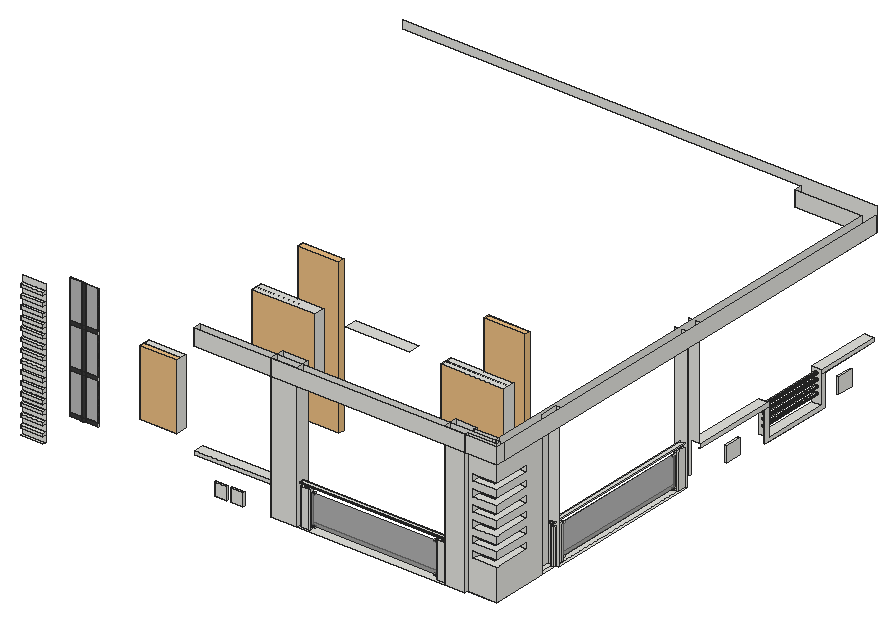
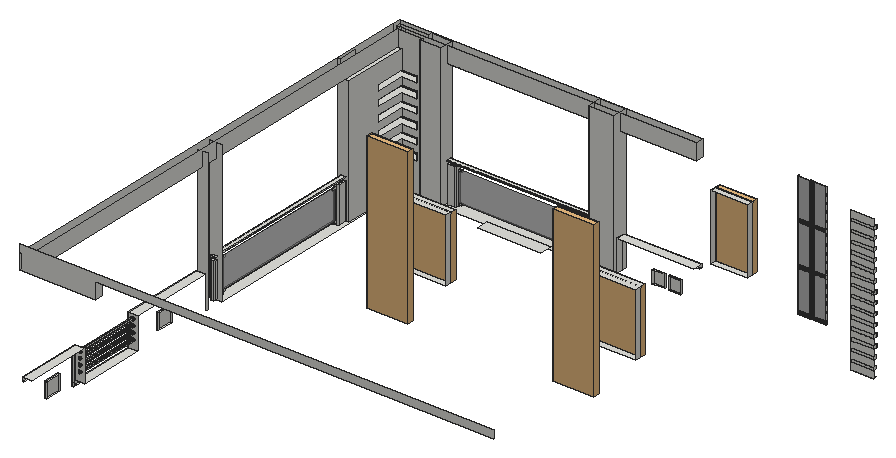
# SketchUp Ruby script. Lengths in inches.
U = 1.inch
M = Sketchup.active_model
def pt(a) = Geom::Point3d.new(a.map { |v| v * U })
def face(e, loops, mat)
  f = e.add_face(loops[0].map { |a| pt(a) })
  loops[1..].each { |l| e.add_face(l.map { |a| pt(a) }).erase! }
  f.material = f.back_material = mat if mat
  f
end
# faces: each face lists its corners as indices into pts; further lists are holes
def faces(e, pts, list, mat = nil) = list.each { |f| face(e, (f[0].is_a?(Array) ? f : [f]).map { |l| l.map { |i| pts[i] } }, mat) }
# xy, xz, yz: faces in a plane at the given z, y or x. An outline is a flat list of corners, or four numbers for a rectangle; further outlines are holes
def ring(l) = l.size == 4 ? [[l[0], l[1]], [l[2], l[1]], [l[2], l[3]], [l[0], l[3]]] : l.each_slice(2).to_a
def flat(e, list, mat, &to3) = list.each { |f| face(e, (f[0].is_a?(Array) ? f : [f]).map { |l| ring(l).map { |u, v| to3.(u, v) } }, mat) }
def xy(e, z, list, mat = nil) = flat(e, list, mat) { |x, y| [x, y, z] }
def xz(e, y, list, mat = nil) = flat(e, list, mat) { |x, z| [x, y, z] }
def yz(e, x, list, mat = nil) = flat(e, list, mat) { |y, z| [x, y, z] }
def lines(e, pts, list) = list.each { |a, b| e.add_line(pt(pts[a]), pt(pts[b])) }
# prism: a flat outline (further loops are holes) pulled along v
def prism(e, loops, v, mat = nil)
  f = face(e, loops, mat); d = Geom::Vector3d.new(v.map { |x| x * U })
  f.pushpull(f.normal.samedirection?(d) ? d.length : -d.length)
end
def box(e, o, s, mat = nil) = prism(e, [[o, [o[0] + s[0], o[1], o[2]], [o[0] + s[0], o[1] + s[1], o[2]], [o[0], o[1] + s[1], o[2]]]], [0, 0, s[2]], mat)
def at(x, y, z, deg = 0) = Geom::Transformation.translation(pt([x, y, z])) * Geom::Transformation.rotation(ORIGIN, Z_AXIS, deg.degrees)
def axes(o, x, y, z) = Geom::Transformation.new([*x, 0, *y, 0, *z, 0, *pt(o).to_a, 1])
def part(name) = M.definitions.add(name)
# library, detail: a bought-in or finely detailed component or shape, given as its bounding box
def library(name, o, s) = part(name).tap { |d| box(d.entities, o, s) }
def detail(e, o, s) = box(e.add_group.entities, o, s)
def put(e, d, t, mat = nil) = e.add_instance(d, t).tap { |i| i.material = mat if mat }
def group(e, t, mat = nil) = e.add_group.tap { |g| g.transformation = t; g.material = mat if mat }.entities
root = M.entities
M.materials.add("[Color M07]").color = [58, 58, 58]
M.materials.add("[Mirror 01]").color = [185, 185, 185]
M.materials.add("[Translucent Glass Gray]").color = [128, 128, 128]
M.materials["[Translucent Glass Gray]"].alpha = 0.5
c1 = library("Curtains 004",[-15.59,-2.26,0],[31.18,4.52,116.91])
c2 = part("Group\#7")
prism(c2.entities,[[[1.18,0.28,0],[1.18,0.28,1.18],[1.18,0.52,1.18],[1.18,0.52,0],[1.18,0.79,0],[1.18,0.79,1.44],[1.18,0,1.44],[1.18,0,0]]],[-1.18,0,0])
c3 = part("Group\#11")
prism(c3.entities,[[[0.44,1.18,0],[0.6,1.2,0],[0.76,1.18,0],[0.9,1.12,0],[1.02,1.02,0],[1.12,0.9,0],[1.18,0.76,0],[1.2,0.6,0],[1.18,0.44,0],[1.12,0.3,0],[1.02,0.18,0],[0.9,0.08,0],[0.76,0.02,0],[0.6,0,0],[0.44,0.02,0],[0.3,0.08,0],[0.18,0.18,0],[0.08,0.3,0],[0.02,0.44,0],[0,0.6,0],[0.02,0.76,0],[0.08,0.9,0],[0.18,1.02,0],[0.3,1.12,0]]],[0,0,2.4])
c4 = part("Group\#1")
prism(c4.entities,[[[0,0.6,0],[0,3,0],[0.6,3.6,0],[3,3.6,0],[3.6,3,0],[3.6,0.6,0],[3,0,0],[0.6,0,0]]],[0,0,36])
c5 = part("Group\#15")
g1 = group(c5.entities,at(0.6,0,38.4))
xy(g1,0,[[-0.6,0.3,51,3.3]])
xy(g1,1.2,[[-0.6,0.3,51,3.3]])
xz(g1,0,[[-0.6,0.3,51,0.9]])
xz(g1,3.6,[[-0.6,0.3,51,0.9]])
yz(g1,-0.6,[[0.3,0,0,0.3,0,0.9,0.3,1.2,3.3,1.2,3.6,0.9,3.6,0.3,3.3,0]])
yz(g1,51,[[0.3,0,3.3,0,3.6,0.3,3.6,0.9,3.3,1.2,0.3,1.2,0,0.9,0,0.3]])
p = [[51,0.3,0],[51,0,0.3],[-0.6,0,0.3],[-0.6,0.3,0],[51,3.6,0.3],[51,3.3,0],
  [-0.6,3.3,0],[-0.6,3.6,0.3],[51,0,0.9],[51,0.3,1.2],[-0.6,0.3,1.2],[-0.6,0,0.9],
  [51,3.3,1.2],[51,3.6,0.9],[-0.6,3.6,0.9],[-0.6,3.3,1.2]]
faces(g1,p,[[0,1,2,3],[4,5,6,7],[8,9,10,11],[12,13,14,15]])
put(c5.entities,c2,at(3.6,1.28,32.42))
put(c5.entities,c2,axes([3.6,1.28,3.58],[1,0,0],[0,1,0],[0,0,-1]))
g2 = group(c5.entities,at(3.6,1.56,0))
box(g2,[0,0,2.4],[44.4,0.24,31.2],"[Translucent Glass Gray]")
g3 = group(c5.entities,at(48,0,0))
put(g3,c3,at(1.2,1.2,36))
put(g3,c4,at(0,0,0))
g4 = group(c5.entities,at(0,0,0))
put(g4,c3,at(1.2,1.2,36))
put(g4,c4,at(0,0,0))
put(c5.entities,c2,axes([46.82,1.28,3.58],[1,0,0],[0,1,0],[0,0,-1]))
put(c5.entities,c2,at(46.82,1.28,32.42))
c6 = part("Glass Ralling")
put(c6.entities,c5,axes([-269.61,-74.06,138],[2.16,0,0],[0,1,0],[0,0,0.75758]))
put(c6.entities,c5,axes([-120.8,-18.44,138],[0,2.4408,0],[-1,0,0],[0,0,0.75758]))
c7 = library("Window 46-10",[-43.56,-2.12,0],[87.13,4.27,82.67])
c8 = library("Window 46-05",[-17.86,-2.78,0],[35.72,4.26,58.96])
xy(root,128.79,[[7.9375,22.625,25.22,25.1875]])
xy(root,133.82,[[7.9375,22.625,25.22,25.1875]])
xy(root,135,[[364.9375,281.83,366.3125,284.83],[364.9375,284.83,366.3125,335.01],[364.9375,335.01,366.3125,338.01]])
xy(root,136.17,[[7.9375,22.625,25.22,25.1875]])
xy(root,136.53,[[151.84,26.8125,161.34,28.1875],[164.22,26.8125,173.72,28.1875]])
xy(root,138,[[196.07,25.625,215.37,28.1875],[215.37,25.625,327.58,36.25],[327.58,25.625,343.4,28.1875],[196.07,28.1875,215.37,34.1875],[327.58,28.1875,359.0625,34.1875],
  [359.0625,28.1875,359.0625,34.1875,358.9375,34.1875,358.9375,84.5,361.9375,84.5,361.9375,28.1875],[361.9375,28.1875,364.9375,84.5],[196.07,34.1875,215.37,36.25],[327.58,34.1875,343.4,36.25],[357.6875,34.1875,358.9375,34.1875,358.9375,84.5,364.9375,84.5,364.9375,206.85,357.6875,206.85],
  [364.9375,84.5,367,206.85],[358.9375,284.83,366.3125,335.01]])
xy(root,138.13,[[364.9375,245.53,366.3125,257.28],[364.9375,351.9,366.3125,363.65]])
xy(root,141.19,[[7.9375,22.625,25.22,25.1875]])
xy(root,143.54,[[7.9375,22.625,25.22,25.1875]])
xy(root,146.03,[[151.84,26.8125,161.34,28.1875],[164.22,26.8125,173.72,28.1875]])
xy(root,148.57,[[7.9375,22.5,25.22,25.1875]])
xy(root,149.88,[[364.9375,245.53,366.3125,257.28],[364.9375,351.9,366.3125,363.65]])
xy(root,150.92,[[7.9375,22.5,25.22,25.1875]])
xy(root,153.17,[[52.28,25.1875,55.28,25.6875],[43.02,25.6875,52.28,26.1875],[52.28,25.6875,55.28,26.1875],[55.28,25.6875,64.8,26.1875]])
xy(root,153.17,[[43.02,25.1875,52.28,25.6875],[55.28,25.1875,64.8,25.6875]],"[Color M07]")
xy(root,155.8,[[52.28,25.1875,55.28,25.6875],[43.02,25.6875,52.28,26.1875],[52.28,25.6875,55.28,26.1875],[55.28,25.6875,64.8,26.1875]])
xy(root,155.8,[[43.02,25.1875,52.28,25.6875],[55.28,25.1875,64.8,25.6875]],"[Color M07]")
xy(root,155.94,[[7.9375,22.5,25.22,25.1875]])
xy(root,158.29,[[7.9375,22.5,25.22,25.1875]])
xy(root,159,[[137.39,26.8125,196.07,28.1875],[364.9375,220.375,366.3125,281.83],[364.9375,338.01,366.3125,385.1875]])
xy(root,161.83,[[347.3125,28.1875,364.9375,28.1875,364.9375,56.8125,358.9375,56.8125,358.9375,34.1875,347.3125,34.1875]])
xy(root,162,[[137.39,26.8125,196.07,34.1875],[94.9375,133.1875,142.9375,142.1875],[238.9375,133.1875,286.9375,142.1875],[358.9375,220.375,366.3125,284.83],[358.9375,335.01,366.3125,385.1875]])
xy(root,163.32,[[7.9375,22.5,25.22,25.1875]])
xy(root,165.67,[[7.9375,22.5,25.22,25.1875]])
xy(root,166.89,[[347.3125,28.1875,358.9375,34.1875],[358.9375,28.1875,364.9375,56.8125]])
xy(root,169.96,[[96.26,25.1875,124.63,34.1875]])
xy(root,170.69,[[7.9375,22.5,25.22,25.1875]])
xy(root,172.33,[[347.3125,28.1875,364.9375,28.1875,364.9375,56.8125,358.9375,56.8125,358.9375,34.1875,347.3125,34.1875]])
xy(root,173.04,[[7.9375,22.5,25.22,25.1875]])
xy(root,177.39,[[347.3125,28.1875,347.3125,34.1875,358.9375,34.1875,358.9375,56.8125,364.9375,56.8125,364.9375,28.1875]])
xy(root,178.07,[[7.9375,22.5,25.22,25.1875]])
xy(root,180.42,[[7.9375,22.5,25.22,25.1875]])
xy(root,182.83,[[347.3125,28.1875,364.9375,28.1875,364.9375,56.8125,358.9375,56.8125,358.9375,34.1875,347.3125,34.1875]])
xy(root,184.48,[[52.28,25.1875,55.28,26.1875],[43.02,25.6875,52.28,26.1875],[55.28,25.6875,64.8,26.1875]])
xy(root,184.48,[[43.02,25.1875,52.28,25.6875],[55.28,25.1875,64.8,25.6875]],"[Color M07]")
xy(root,185.44,[[7.9375,22.5,25.22,25.0625],[7.9375,25.0625,25.22,25.1875]])
xy(root,187.11,[[52.28,25.1875,55.28,26.1875],[43.02,25.6875,52.28,26.1875],[55.28,25.6875,64.8,26.1875]])
xy(root,187.11,[[43.02,25.1875,52.28,25.6875],[55.28,25.1875,64.8,25.6875]],"[Color M07]")
xy(root,187.79,[[7.9375,22.5,25.22,25.0625],[7.9375,25.0625,25.22,25.1875]])
xy(root,187.89,[[347.3125,28.1875,347.3125,34.1875,358.9375,34.1875,358.9375,56.8125,364.9375,56.8125,364.9375,28.1875]])
xy(root,192.82,[[7.9375,22.625,25.22,25.1875]])
xy(root,193.33,[[347.3125,28.1875,364.9375,28.1875,364.9375,56.8125,358.9375,56.8125,358.9375,34.1875,347.3125,34.1875]])
xy(root,195.17,[[7.9375,22.625,25.22,25.1875]])
xy(root,198.39,[[347.3125,28.1875,347.3125,34.1875,358.9375,34.1875,358.9375,56.8125,364.9375,56.8125,364.9375,28.1875]])
xy(root,200.19,[[7.9375,22.625,25.22,25.1875]])
xy(root,202.54,[[7.9375,22.625,25.22,25.1875]])
xy(root,203.83,[[347.3125,28.1875,364.9375,28.1875,364.9375,56.8125,358.9375,56.8125,358.9375,34.1875,347.3125,34.1875]])
xy(root,207.57,[[7.9375,22.625,25.22,25.1875]])
xy(root,208.89,[[347.3125,28.1875,347.3125,34.1875,358.9375,34.1875,358.9375,56.8125,364.9375,56.8125,364.9375,28.1875]])
xy(root,209.92,[[7.9375,22.625,25.22,25.1875]])
xy(root,210,[[94.9375,133.1875,142.9375,142.1875],[166.9375,133.1875,214.9375,142.1875],[238.9375,133.1875,286.9375,142.1875]])
xy(root,214.33,[[347.3125,28.1875,364.9375,28.1875,364.9375,56.8125,358.9375,56.8125,358.9375,34.1875,347.3125,34.1875]])
xy(root,214.94,[[7.9375,22.625,25.22,25.1875]])
xy(root,215.79,[[52.28,25.1875,55.28,26.1875],[43.02,25.6875,52.28,26.1875],[55.28,25.6875,64.8,26.1875]])
xy(root,215.79,[[43.02,25.1875,52.28,25.6875],[55.28,25.1875,64.8,25.6875]],"[Color M07]")
xy(root,217.29,[[7.9375,22.625,25.22,25.1875]])
xy(root,218.42,[[52.28,25.1875,55.28,26.1875],[43.02,25.6875,52.28,26.1875],[55.28,25.6875,64.8,26.1875]])
xy(root,218.42,[[43.02,25.1875,52.28,25.6875],[55.28,25.1875,64.8,25.6875]],"[Color M07]")
xy(root,219.39,[[347.3125,28.1875,347.3125,34.1875,358.9375,34.1875,358.9375,56.8125,364.9375,56.8125,364.9375,28.1875]])
xy(root,219.71,[[96.26,25.1875,124.63,34.1875]])
xy(root,222.32,[[7.9375,22.625,25.22,25.1875]])
xy(root,224.67,[[7.9375,22.625,25.22,25.1875]])
xy(root,229.69,[[7.9375,22.5,25.22,25.1875]])
xy(root,232.04,[[7.9375,22.5,25.22,25.1875]])
xy(root,234,[[137.39,25.1875,367.9375,31.1875],[359.0625,31.1875,361.9375,34.1875],[361.9375,31.1875,364.9375,84.5],[364.9375,31.1875,364.9375,84.5,361.9375,84.5,361.9375,385.1875,367.9375,385.1875,367.9375,31.1875],[358.9375,34.1875,361.9375,84.5],
  [310.9375,379.1875,361.9375,385.1875]])
xz(root,22.5,[[7.9375,148.57,25.22,150.92],[7.9375,155.94,25.22,158.29],[7.9375,163.32,25.22,165.67],[7.9375,170.69,25.22,173.04],[7.9375,178.07,25.22,180.42],
  [7.9375,185.44,25.22,187.79],[7.9375,229.69,25.22,232.04]])
xz(root,22.625,[[7.9375,133.82,25.22,136.17],[7.9375,141.19,25.22,143.54],[7.9375,192.82,25.22,195.17],[7.9375,200.19,25.22,202.54],[7.9375,207.57,25.22,209.92],
  [7.9375,214.94,25.22,217.29],[7.9375,222.32,25.22,224.67]])
xz(root,25.0625,[[7.9375,185.44,25.22,187.79]])
xz(root,25.1875,[[7.9375,128.79,25.22,133.82],[7.9375,133.82,25.22,136.17],[7.9375,136.17,25.22,141.19],[7.9375,141.19,25.22,143.54],[7.9375,143.54,25.22,148.57],
  [7.9375,148.57,25.22,150.92],[7.9375,150.92,25.22,155.94],[7.9375,155.94,25.22,158.29],[7.9375,158.29,25.22,163.32],[7.9375,163.32,25.22,165.67],
  [7.9375,165.67,25.22,170.69],[7.9375,170.69,25.22,173.04],[7.9375,173.04,25.22,178.07],[7.9375,178.07,25.22,180.42],[7.9375,180.42,25.22,185.44],
  [7.9375,185.44,25.22,187.79],[7.9375,187.79,25.22,192.82],[7.9375,192.82,25.22,195.17],[7.9375,195.17,25.22,200.19],[7.9375,200.19,25.22,202.54],
  [7.9375,202.54,25.22,207.57],[7.9375,207.57,25.22,209.92],[7.9375,209.92,25.22,214.94],[7.9375,214.94,25.22,217.29],[7.9375,217.29,25.22,222.32],
  [7.9375,222.32,25.22,224.67],[7.9375,224.67,25.22,229.69],[7.9375,229.69,25.22,232.04],[7.9375,232.04,25.22,237.07],[137.39,234,367.9375,246]])
xz(root,25.1875,[[43.02,153.17,52.28,155.8],[52.28,153.17,55.28,155.8],[55.28,153.17,64.8,155.8],[52.28,155.8,55.28,184.48],[43.02,184.48,52.28,187.11],
  [52.28,184.48,55.28,187.11],[55.28,184.48,64.8,187.11],[52.28,187.11,55.28,215.79],[43.02,215.79,52.28,218.42],[52.28,215.79,55.28,218.42],
  [55.28,215.79,64.8,218.42],[52.28,218.42,55.28,247.11]],"[Color M07]")
xz(root,25.625,[[196.07,138,215.37,246],[327.58,138,343.4,246]])
xz(root,25.6875,[[43.02,153.17,52.28,155.8],[52.28,153.17,55.28,155.8],[55.28,153.17,64.8,155.8]])
xz(root,25.6875,[[43.02,155.8,52.28,184.48],[55.28,155.8,64.8,184.48],[43.02,187.11,52.28,215.79],[55.28,187.11,64.8,215.79],[43.02,218.42,52.28,247.11],
  [55.28,218.42,64.8,247.11]],"[Mirror 01]")
xz(root,26.1875,[[43.02,153.17,52.28,155.8],[52.28,153.17,55.28,155.8],[55.28,153.17,64.8,155.8],[52.28,155.8,55.28,184.48],[43.02,184.48,52.28,187.11],
  [52.28,184.48,55.28,187.11],[55.28,184.48,64.8,187.11],[52.28,187.11,55.28,215.79],[43.02,215.79,52.28,218.42],[52.28,215.79,55.28,218.42],
  [55.28,215.79,64.8,218.42],[52.28,218.42,55.28,247.11]],"[Color M07]")
xz(root,26.1875,[[43.02,155.8,52.28,184.48],[55.28,155.8,64.8,184.48],[43.02,187.11,52.28,215.79],[55.28,187.11,64.8,215.79],[43.02,218.42,52.28,247.11],
  [55.28,218.42,64.8,247.11]],"[Mirror 01]")
xz(root,26.8125,[[151.84,136.53,161.34,146.03],[164.22,136.53,173.72,146.03],[137.39,159,196.07,162]])
xz(root,28.1875,[[343.4,138,364.9375,138,364.9375,161.83,347.3125,161.83,347.3125,166.89,364.9375,166.89,364.9375,172.33,347.3125,172.33,347.3125,177.39,364.9375,177.39,364.9375,182.83,347.3125,182.83,347.3125,187.89,364.9375,187.89,364.9375,193.33,347.3125,193.33,347.3125,198.39,364.9375,198.39,364.9375,203.83,347.3125,203.83,347.3125,208.89,364.9375,208.89,364.9375,214.33,347.3125,214.33,347.3125,219.39,364.9375,219.39,364.9375,246,343.4,246]])
xz(root,31.1875,[[137.39,234,359.0625,246],[359.0625,234,361.9375,246],[361.9375,234,364.9375,246]])
xz(root,34.1875,[[343.4,138,343.4,246,361.9375,246,361.9375,234,358.9375,234,358.9375,219.39,347.3125,219.39,347.3125,214.33,358.9375,214.33,358.9375,208.89,347.3125,208.89,347.3125,203.83,358.9375,203.83,358.9375,198.39,347.3125,198.39,347.3125,193.33,358.9375,193.33,358.9375,187.89,347.3125,187.89,347.3125,182.83,358.9375,182.83,358.9375,177.39,347.3125,177.39,347.3125,172.33,358.9375,172.33,358.9375,166.89,347.3125,166.89,347.3125,161.83,358.9375,161.83,358.9375,138]])
xz(root,36.25,[[196.07,138,215.37,246],[327.58,138,343.4,246]])
xz(root,56.8125,[[358.9375,161.83,364.9375,166.89],[358.9375,172.33,364.9375,177.39],[358.9375,182.83,364.9375,187.89],[358.9375,193.33,364.9375,198.39],[358.9375,203.83,364.9375,208.89],
  [358.9375,214.33,364.9375,219.39]])
xz(root,84.5,[[358.9375,138,358.9375,234,364.9375,234,364.9375,247,367,247,367,138]])
xz(root,206.85,[[357.6875,138,367,244.8125]])
xz(root,220.375,[[357.6875,138,357.6875,244.8125,364.9375,244.8125,364.9375,162,358.9375,162,358.9375,138]])
xz(root,245.53,[[364.9375,138.13,366.3125,149.88]])
xz(root,257.28,[[364.9375,138.13,366.3125,149.88]])
xz(root,281.83,[[364.9375,135,366.3125,138],[364.9375,138,366.3125,159]])
xz(root,284.83,[[[358.9375,138,366.3125,162],[362.59,157.69,362.88,157.73,363.16,157.84,363.39,158.01,363.57,158.24,363.6875,158.52,363.73,158.81,363.69,159.1,363.58,159.37,363.4,159.6,363.17,159.79,362.9,159.9,362.61,159.94,362.32,159.91,362.05,159.8,361.8125,159.62,361.63,159.39,361.52,159.12,361.48,158.83,361.51,158.54,361.62,158.26,361.8,158.03,362.03,157.85,362.3,157.73],[362.59,153,362.88,153.04,363.16,153.15,363.39,153.33,363.57,153.56,363.6875,153.83,363.73,154.12,363.69,154.41,363.58,154.68,363.4,154.92,363.17,155.1,362.9,155.21,362.61,155.25,362.32,155.22,362.05,155.11,361.8125,154.93,361.63,154.7,361.52,154.43,361.48,154.14,361.51,153.85,361.62,153.58,361.8,153.34,362.03,153.16,362.3,153.05],[362.59,148.32,362.88,148.35,363.16,148.46,363.39,148.64,363.57,148.87,363.6875,149.14,363.73,149.43,363.69,149.72,363.58,149.99,363.4,150.23,363.17,150.41,362.9,150.53,362.61,150.57,362.32,150.53,362.05,150.42,361.8125,150.24,361.63,150.01,361.52,149.74,361.48,149.45,361.51,149.16,361.62,148.89,361.8,148.65,362.03,148.47,362.3,148.36],[362.59,143.63,362.88,143.66,363.16,143.77,363.39,143.95,363.57,144.18,363.6875,144.45,363.73,144.74,363.69,145.03,363.58,145.31,363.4,145.54,363.17,145.72,362.9,145.84,362.61,145.88,362.32,145.84,362.05,145.73,361.8125,145.56,361.63,145.33,361.52,145.06,361.48,144.76,361.51,144.47,361.62,144.2,361.8,143.97,362.03,143.78,362.3,143.67]]])
xz(root,335.01,[[[358.9375,138,366.3125,162],[362.59,153,362.3,153.05,362.03,153.16,361.8,153.34,361.62,153.58,361.51,153.85,361.48,154.14,361.52,154.43,361.63,154.7,361.8125,154.93,362.05,155.11,362.32,155.22,362.61,155.25,362.9,155.21,363.17,155.1,363.4,154.92,363.58,154.68,363.69,154.41,363.73,154.12,363.6875,153.83,363.57,153.56,363.39,153.33,363.16,153.15,362.88,153.04],[362.59,148.32,362.3,148.36,362.03,148.47,361.8,148.65,361.62,148.89,361.51,149.16,361.48,149.45,361.52,149.74,361.63,150.01,361.8125,150.24,362.05,150.42,362.32,150.53,362.61,150.57,362.9,150.53,363.17,150.41,363.4,150.23,363.58,149.99,363.69,149.72,363.73,149.43,363.6875,149.14,363.57,148.87,363.39,148.64,363.16,148.46,362.88,148.35],[362.59,143.63,362.3,143.67,362.03,143.78,361.8,143.97,361.62,144.2,361.51,144.47,361.48,144.76,361.52,145.06,361.63,145.33,361.8125,145.56,362.05,145.73,362.32,145.84,362.61,145.88,362.9,145.84,363.17,145.72,363.4,145.54,363.58,145.31,363.69,145.03,363.73,144.74,363.6875,144.45,363.57,144.18,363.39,143.95,363.16,143.77,362.88,143.66],[362.59,157.69,362.3,157.73,362.03,157.85,361.8,158.03,361.62,158.26,361.51,158.54,361.48,158.83,361.52,159.12,361.63,159.39,361.8125,159.62,362.05,159.8,362.32,159.91,362.61,159.94,362.9,159.9,363.17,159.79,363.4,159.6,363.58,159.37,363.69,159.1,363.73,158.81,363.6875,158.52,363.57,158.24,363.39,158.01,363.16,157.84,362.88,157.73]]])
xz(root,338.01,[[364.9375,135,366.3125,138],[364.9375,138,366.3125,159]])
xz(root,351.9,[[364.9375,138.13,366.3125,149.88]])
xz(root,363.65,[[364.9375,138.13,366.3125,149.88]])
xz(root,379.1875,[[310.9375,234,361.9375,246]])
xz(root,385.1875,[[310.9375,234,310.9375,246,7.9375,246,7.9375,252,367.9375,252,367.9375,234]])
yz(root,7.9375,[[22.625,133.82,25.1875,136.17],[22.625,141.19,25.1875,143.54],[22.5,148.57,25.1875,150.92],[22.5,155.94,25.1875,158.29],[22.5,163.32,25.1875,165.67],
  [22.5,170.69,25.1875,173.04],[22.5,178.07,25.1875,180.42],[22.5,185.44,25.0625,187.79],[25.0625,185.44,25.1875,187.79],[22.625,192.82,25.1875,195.17],
  [22.625,200.19,25.1875,202.54],[22.625,207.57,25.1875,209.92],[22.625,214.94,25.1875,217.29],[22.625,222.32,25.1875,224.67],[22.5,229.69,25.1875,232.04]])
yz(root,25.22,[[22.625,133.82,25.1875,136.17],[22.625,141.19,25.1875,143.54],[22.5,148.57,25.1875,150.92],[22.5,155.94,25.1875,158.29],[22.5,163.32,25.1875,165.67],
  [22.5,170.69,25.1875,173.04],[22.5,178.07,25.1875,180.42],[22.5,185.44,25.0625,187.79],[25.0625,185.44,25.1875,187.79],[22.625,192.82,25.1875,195.17],
  [22.625,200.19,25.1875,202.54],[22.625,207.57,25.1875,209.92],[22.625,214.94,25.1875,217.29],[22.625,222.32,25.1875,224.67],[22.5,229.69,25.1875,232.04]])
yz(root,43.02,[[25.1875,153.17,25.6875,155.8],[25.6875,153.17,26.1875,155.8],[25.6875,155.8,26.1875,184.48],[25.1875,184.48,26.1875,187.11],[25.6875,187.11,26.1875,215.79],
  [25.1875,215.79,26.1875,218.42],[25.6875,218.42,26.1875,247.11]])
yz(root,43.02,[[25.1875,155.8,25.6875,184.48],[25.1875,187.11,25.6875,215.79],[25.1875,218.42,25.6875,247.11]],"[Color M07]")
yz(root,52.28,[[25.1875,153.17,25.6875,155.8],[25.6875,153.17,26.1875,155.8],[25.6875,155.8,26.1875,184.48],[25.1875,184.48,26.1875,187.11],[25.6875,187.11,26.1875,215.79],
  [25.1875,215.79,26.1875,218.42],[25.6875,218.42,26.1875,247.11]])
yz(root,52.28,[[25.1875,155.8,25.6875,184.48],[25.1875,187.11,25.6875,215.79],[25.1875,218.42,25.6875,247.11]],"[Color M07]")
yz(root,55.28,[[25.1875,153.17,25.6875,155.8],[25.6875,153.17,26.1875,155.8],[25.6875,155.8,26.1875,184.48],[25.1875,184.48,26.1875,187.11],[25.6875,187.11,26.1875,215.79],
  [25.1875,215.79,26.1875,218.42],[25.6875,218.42,26.1875,247.11]])
yz(root,55.28,[[25.1875,155.8,25.6875,184.48],[25.1875,187.11,25.6875,215.79],[25.1875,218.42,25.6875,247.11]],"[Color M07]")
yz(root,64.8,[[25.1875,153.17,25.6875,155.8],[25.6875,153.17,26.1875,155.8],[25.6875,155.8,26.1875,184.48],[25.1875,184.48,26.1875,187.11],[25.6875,187.11,26.1875,215.79],
  [25.1875,215.79,26.1875,218.42],[25.6875,218.42,26.1875,247.11]])
yz(root,64.8,[[25.1875,155.8,25.6875,184.48],[25.1875,187.11,25.6875,215.79],[25.1875,218.42,25.6875,247.11]],"[Color M07]")
yz(root,94.9375,[[133.1875,162,142.1875,210]])
yz(root,96.26,[[25.1875,169.96,34.1875,219.71]])
yz(root,124.63,[[25.1875,169.96,34.1875,219.71]])
yz(root,137.39,[[25.1875,234,31.1875,246]])
yz(root,142.9375,[[133.1875,162,142.1875,210]])
yz(root,151.84,[[26.8125,136.53,28.1875,146.03]])
yz(root,161.34,[[26.8125,136.53,28.1875,146.03]])
yz(root,164.22,[[26.8125,136.53,28.1875,146.03]])
yz(root,173.72,[[26.8125,136.53,28.1875,146.03]])
yz(root,196.07,[[25.625,138,25.625,246,36.25,246,36.25,138,34.1875,138,34.1875,162,26.8125,162,26.8125,159,28.1875,159,28.1875,138],[28.1875,138,28.1875,159,26.8125,159,26.8125,162,34.1875,162,34.1875,138]])
yz(root,215.37,[[25.625,138,36.25,246]])
yz(root,238.9375,[[133.1875,162,142.1875,210]])
yz(root,286.9375,[[133.1875,162,142.1875,210]])
yz(root,310.9375,[[379.1875,234,385.1875,246]])
yz(root,327.58,[[25.625,138,36.25,246]])
yz(root,343.4,[[25.625,138,28.1875,246],[34.1875,138,36.25,246]])
yz(root,347.3125,[[28.1875,161.83,34.1875,166.89],[28.1875,172.33,34.1875,177.39],[28.1875,182.83,34.1875,187.89],[28.1875,193.33,34.1875,198.39],[28.1875,203.83,34.1875,208.89],
  [28.1875,214.33,34.1875,219.39]])
yz(root,358.9375,[[34.1875,138,34.1875,161.83,56.8125,161.83,56.8125,166.89,34.1875,166.89,34.1875,172.33,56.8125,172.33,56.8125,177.39,34.1875,177.39,34.1875,182.83,56.8125,182.83,56.8125,187.89,34.1875,187.89,34.1875,193.33,56.8125,193.33,56.8125,198.39,34.1875,198.39,34.1875,203.83,56.8125,203.83,56.8125,208.89,34.1875,208.89,34.1875,214.33,56.8125,214.33,56.8125,219.39,34.1875,219.39,34.1875,234,84.5,234,84.5,138]])
yz(root,361.9375,[[31.1875,234,34.1875,246],[34.1875,234,379.1875,246]])
yz(root,364.9375,[[28.1875,138,70.91,138,70.91,234,31.1875,234,31.1875,246,28.1875,246,28.1875,219.39,56.8125,219.39,56.8125,214.33,28.1875,214.33,28.1875,208.89,56.8125,208.89,56.8125,203.83,28.1875,203.83,28.1875,198.39,56.8125,198.39,56.8125,193.33,28.1875,193.33,28.1875,187.89,56.8125,187.89,56.8125,182.83,28.1875,182.83,28.1875,177.39,56.8125,177.39,56.8125,172.33,28.1875,172.33,28.1875,166.89,56.8125,166.89,56.8125,161.83,28.1875,161.83],[70.91,234,84.5,247]])
yz(root,366.3125,[[281.83,135,338.01,135,338.01,159,335.01,159,335.01,138,284.83,138,284.83,159,281.83,159],[245.53,138.13,257.28,149.88],[351.9,138.13,363.65,149.88],[220.375,159,284.83,162],[335.01,159,385.1875,162]])
yz(root,367.9375,[[25.1875,234,31.1875,246],[31.1875,234,385.1875,246]])
p = [[362.3,335.01,143.67],[362.59,335.01,143.63],[362.59,284.83,143.63],[362.3,284.83,143.67],[362.88,335.01,143.66],[362.88,284.83,143.66],
  [362.03,335.01,143.78],[362.03,284.83,143.78],[363.16,335.01,143.77],[363.16,284.83,143.77],[361.8,335.01,143.97],[361.8,284.83,143.97],
  [363.39,335.01,143.95],[363.39,284.83,143.95],[361.62,335.01,144.2],[361.62,284.83,144.2],[363.57,335.01,144.18],[363.57,284.83,144.18],
  [361.51,335.01,144.47],[361.51,284.83,144.47],[363.6875,335.01,144.45],[363.6875,284.83,144.45],[361.48,335.01,144.76],[361.48,284.83,144.76],
  [363.73,335.01,144.74],[363.73,284.83,144.74],[363.69,335.01,145.03],[363.69,284.83,145.03],[361.52,335.01,145.06],[361.52,284.83,145.06],
  [363.58,335.01,145.31],[363.58,284.83,145.31],[361.63,335.01,145.33],[361.63,284.83,145.33],[361.8125,335.01,145.56],[361.8125,284.83,145.56],
  [363.4,335.01,145.54],[363.4,284.83,145.54],[363.17,335.01,145.72],[363.17,284.83,145.72],[362.05,335.01,145.73],[362.05,284.83,145.73],
  [362.32,335.01,145.84],[362.32,284.83,145.84],[362.9,335.01,145.84],[362.9,284.83,145.84],[362.61,335.01,145.88],[362.61,284.83,145.88],
  [362.3,335.01,148.36],[362.59,335.01,148.32],[362.59,284.83,148.32],[362.3,284.83,148.36],[362.88,335.01,148.35],[362.88,284.83,148.35],
  [362.03,335.01,148.47],[362.03,284.83,148.47],[363.16,335.01,148.46],[363.16,284.83,148.46],[361.8,335.01,148.65],[361.8,284.83,148.65],
  [363.39,335.01,148.64],[363.39,284.83,148.64],[363.57,335.01,148.87],[363.57,284.83,148.87],[361.62,335.01,148.89],[361.62,284.83,148.89],
  [361.51,335.01,149.16],[361.51,284.83,149.16],[363.6875,335.01,149.14],[363.6875,284.83,149.14],[363.73,335.01,149.43],[363.73,284.83,149.43],
  [361.48,335.01,149.45],[361.48,284.83,149.45],[363.69,335.01,149.72],[363.69,284.83,149.72],[361.52,335.01,149.74],[361.52,284.83,149.74],
  [361.63,335.01,150.01],[361.63,284.83,150.01],[363.58,335.01,149.99],[363.58,284.83,149.99],[361.8125,335.01,150.24],[361.8125,284.83,150.24],
  [363.4,335.01,150.23],[363.4,284.83,150.23],[362.05,335.01,150.42],[362.05,284.83,150.42],[363.17,335.01,150.41],[363.17,284.83,150.41],
  [362.32,335.01,150.53],[362.32,284.83,150.53],[362.9,335.01,150.53],[362.9,284.83,150.53],[362.61,335.01,150.57],[362.61,284.83,150.57],
  [362.03,335.01,153.16],[362.3,335.01,153.05],[362.3,284.83,153.05],[362.03,284.83,153.16],[362.59,335.01,153],[362.59,284.83,153],
  [362.88,335.01,153.04],[362.88,284.83,153.04],[363.16,335.01,153.15],[363.16,284.83,153.15],[363.39,335.01,153.33],[363.39,284.83,153.33],
  [361.8,335.01,153.34],[361.8,284.83,153.34],[361.62,335.01,153.58],[361.62,284.83,153.58],[363.57,335.01,153.56],[363.57,284.83,153.56],
  [361.51,335.01,153.85],[361.51,284.83,153.85],[363.6875,335.01,153.83],[363.6875,284.83,153.83],[361.48,335.01,154.14],[361.48,284.83,154.14],
  [363.73,335.01,154.12],[363.73,284.83,154.12],[361.52,335.01,154.43],[361.52,284.83,154.43],[363.69,335.01,154.41],[363.69,284.83,154.41],
  [361.63,335.01,154.7],[361.63,284.83,154.7],[363.58,335.01,154.68],[363.58,284.83,154.68],[361.8125,335.01,154.93],[361.8125,284.83,154.93],
  [363.4,335.01,154.92],[363.4,284.83,154.92],[362.05,335.01,155.11],[362.05,284.83,155.11],[363.17,335.01,155.1],[363.17,284.83,155.1],
  [362.32,335.01,155.22],[362.32,284.83,155.22],[362.9,335.01,155.21],[362.9,284.83,155.21],[362.61,335.01,155.25],[362.61,284.83,155.25],
  [362.03,335.01,157.85],[362.3,335.01,157.73],[362.3,284.83,157.73],[362.03,284.83,157.85],[362.59,335.01,157.69],[362.59,284.83,157.69],
  [362.88,335.01,157.73],[362.88,284.83,157.73],[363.16,335.01,157.84],[363.16,284.83,157.84],[361.8,335.01,158.03],[361.8,284.83,158.03],
  [363.39,335.01,158.01],[363.39,284.83,158.01],[361.62,335.01,158.26],[361.62,284.83,158.26],[363.57,335.01,158.24],[363.57,284.83,158.24],
  [363.6875,335.01,158.52],[363.6875,284.83,158.52],[361.51,335.01,158.54],[361.51,284.83,158.54],[361.48,335.01,158.83],[361.48,284.83,158.83],
  [363.73,335.01,158.81],[363.73,284.83,158.81],[361.52,335.01,159.12],[361.52,284.83,159.12],[363.69,335.01,159.1],[363.69,284.83,159.1],
  [361.63,335.01,159.39],[361.63,284.83,159.39],[363.58,335.01,159.37],[363.58,284.83,159.37],[361.8125,335.01,159.62],[361.8125,284.83,159.62],
  [363.4,335.01,159.6],[363.4,284.83,159.6],[362.05,335.01,159.8],[362.05,284.83,159.8],[363.17,335.01,159.79],[363.17,284.83,159.79],
  [362.32,335.01,159.91],[362.32,284.83,159.91],[362.9,335.01,159.9],[362.9,284.83,159.9],[362.61,335.01,159.94],[362.61,284.83,159.94]]
faces(root,p,[[0,1,2,3],[1,4,5,2],[6,0,3,7],[4,8,9,5],[10,6,7,11],[8,12,13,9],[14,10,11,15],[12,16,17,13],
  [18,14,15,19],[16,20,21,17],[22,18,19,23],[20,24,25,21],[24,26,27,25],[28,22,23,29],[26,30,31,27],[32,28,29,33],
  [34,32,33,35],[30,36,37,31],[36,38,39,37],[40,34,35,41],[42,40,41,43],[38,44,45,39],[46,42,43,47],[44,46,47,45],
  [48,49,50,51],[49,52,53,50],[54,48,51,55],[52,56,57,53],[58,54,55,59],[56,60,61,57],[60,62,63,61],[64,58,59,65],
  [66,64,65,67],[62,68,69,63],[68,70,71,69],[72,66,67,73],[70,74,75,71],[76,72,73,77],[78,76,77,79],[74,80,81,75],
  [82,78,79,83],[80,84,85,81],[86,82,83,87],[84,88,89,85],[90,86,87,91],[88,92,93,89],[94,90,91,95],[92,94,95,93],
  [96,97,98,99],[97,100,101,98],[100,102,103,101],[102,104,105,103],[104,106,107,105],[108,96,99,109],[110,108,109,111],[106,112,113,107],
  [114,110,111,115],[112,116,117,113],[118,114,115,119],[116,120,121,117],[122,118,119,123],[120,124,125,121],[126,122,123,127],[124,128,129,125],
  [130,126,127,131],[128,132,133,129],[134,130,131,135],[132,136,137,133],[138,134,135,139],[136,140,141,137],[142,138,139,143],[140,142,143,141],
  [144,145,146,147],[145,148,149,146],[148,150,151,149],[150,152,153,151],[154,144,147,155],[152,156,157,153],[158,154,155,159],[156,160,161,157],
  [160,162,163,161],[164,158,159,165],[166,164,165,167],[162,168,169,163],[170,166,167,171],[168,172,173,169],[174,170,171,175],[172,176,177,173],
  [178,174,175,179],[176,180,181,177],[182,178,179,183],[180,184,185,181],[186,182,183,187],[184,188,189,185],[190,186,187,191],[188,190,191,189]])
put(root,c1,at(279.9,144.45,129.09))
put(root,c1,at(138.86,144.45,129.09))
put(root,c6,at(485.74,101.65,0))
put(root,c7,axes([118.93,135.31,162],[0.5509,0,0],[0,1,0],[0,0,0.58062]))
put(root,c7,axes([262.93,135.31,162],[0.5509,0,0],[0,1,0],[0,0,0.58062]))
put(root,c8,axes([110.44,27.97,169.96],[0.79416,0,0],[0,1,0],[0,0,0.84382]))
